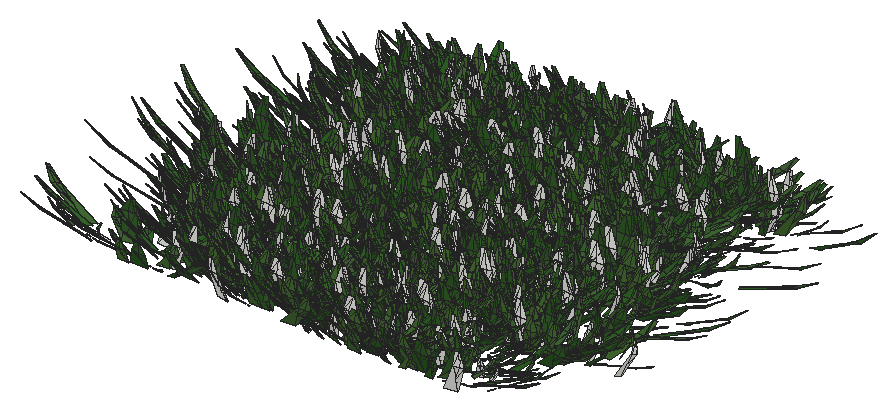
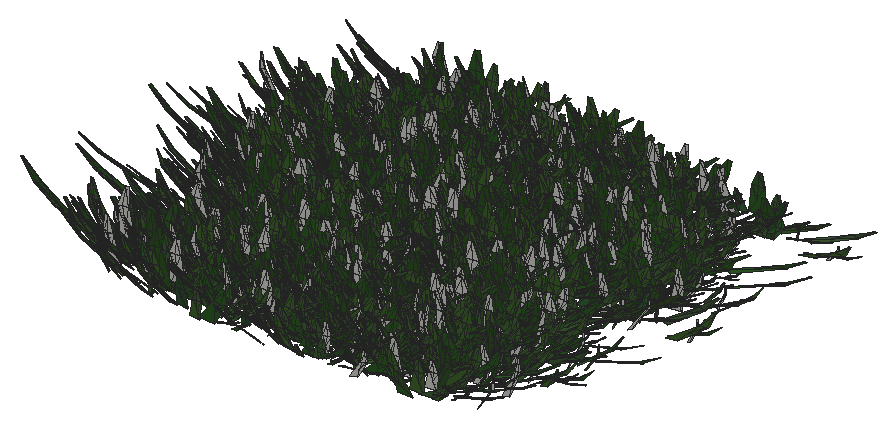
# SketchUp Ruby script. Lengths in inches.
U = 1.inch
M = Sketchup.active_model
def pt(a) = Geom::Point3d.new(a.map { |v| v * U })
def face(e, loops, mat)
  f = e.add_face(loops[0].map { |a| pt(a) })
  loops[1..].each { |l| e.add_face(l.map { |a| pt(a) }).erase! }
  f.material = f.back_material = mat if mat
  f
end
# faces: each face lists its corners as indices into pts; further lists are holes
def faces(e, pts, list, mat = nil) = list.each { |f| face(e, (f[0].is_a?(Array) ? f : [f]).map { |l| l.map { |i| pts[i] } }, mat) }
# xy, xz, yz: faces in a plane at the given z, y or x. An outline is a flat list of corners, or four numbers for a rectangle; further outlines are holes
def ring(l) = l.size == 4 ? [[l[0], l[1]], [l[2], l[1]], [l[2], l[3]], [l[0], l[3]]] : l.each_slice(2).to_a
def flat(e, list, mat, &to3) = list.each { |f| face(e, (f[0].is_a?(Array) ? f : [f]).map { |l| ring(l).map { |u, v| to3.(u, v) } }, mat) }
def xy(e, z, list, mat = nil) = flat(e, list, mat) { |x, y| [x, y, z] }
def xz(e, y, list, mat = nil) = flat(e, list, mat) { |x, z| [x, y, z] }
def yz(e, x, list, mat = nil) = flat(e, list, mat) { |y, z| [x, y, z] }
def lines(e, pts, list) = list.each { |a, b| e.add_line(pt(pts[a]), pt(pts[b])) }
# prism: a flat outline (further loops are holes) pulled along v
def prism(e, loops, v, mat = nil)
  f = face(e, loops, mat); d = Geom::Vector3d.new(v.map { |x| x * U })
  f.pushpull(f.normal.samedirection?(d) ? d.length : -d.length)
end
def box(e, o, s, mat = nil) = prism(e, [[o, [o[0] + s[0], o[1], o[2]], [o[0] + s[0], o[1] + s[1], o[2]], [o[0], o[1] + s[1], o[2]]]], [0, 0, s[2]], mat)
def at(x, y, z, deg = 0) = Geom::Transformation.translation(pt([x, y, z])) * Geom::Transformation.rotation(ORIGIN, Z_AXIS, deg.degrees)
def axes(o, x, y, z) = Geom::Transformation.new([*x, 0, *y, 0, *z, 0, *pt(o).to_a, 1])
def part(name) = M.definitions.add(name)
# library, detail: a bought-in or finely detailed component or shape, given as its bounding box
def library(name, o, s) = part(name).tap { |d| box(d.entities, o, s) }
def detail(e, o, s) = box(e.add_group.entities, o, s)
def put(e, d, t, mat = nil) = e.add_instance(d, t).tap { |i| i.material = mat if mat }
def group(e, t, mat = nil) = e.add_group.tap { |g| g.transformation = t; g.material = mat if mat }.entities
root = M.entities
M.materials.add("Material10").color = [48, 100, 38]
M.materials.add("Material3").color = [68, 110, 58]
M.materials.add("Material4").color = [48, 90, 38]
M.materials.add("Material5").color = [68, 110, 48]
M.materials.add("Material6").color = [48, 90, 48]
M.materials.add("Material7").color = [58, 110, 58]
M.materials.add("Material8").color = [58, 90, 38]
M.materials.add("Material9").color = [68, 100, 58]
c1 = part("grass00")
p = [[-0.6875,0.15,0],[-0.56,0.08,5.52],[-0.04,0.03,2.76],[0.48,-0.02,0],[0.35,-0.02,5.52],[-0.1,-0.14,5.52],
  [-0.12,0.65,8.37],[-0.42,0.65,8.37]]
faces(c1.entities,p,[[0,1,2,3],[3,2,4],[1,5,2],[5,4,2],[1,6,5],[4,5,6],[7,6,1]])
c2 = part("Group16\#1")
put(c2.entities,c1,axes([1.44,-0.61,-0.01],[0.05352,0.12609,0],[-0.10704,0.04543,0.07239],[0.06664,-0.02828,0.11628]),"Material6")
put(c2.entities,c1,axes([0.76,-0.15,-0.01],[0.04676,0.24062,0],[-0.23162,0.04501,0.06642],[0.0652,-0.01267,0.23595]),"Material3")
put(c2.entities,c1,axes([0.79,0.01,-0.01],[-0.00606,0.34651,0],[-0.34381,-0.00602,0.0432],[0.04319,0.00076,0.34386]))
put(c2.entities,c1,axes([1,0.23,-0.01],[-0.07192,0.31144,0],[-0.28722,-0.06632,0.1236],[0.12043,0.02781,0.29478]),"Material5")
put(c2.entities,c1,axes([1.66,0.77,-0.01],[-0.13828,0.29651,0],[-0.21551,-0.1005,0.22471],[0.20365,0.09498,0.23779]),"Material10")
put(c2.entities,c1,axes([0.6875,0.52,-0.01],[-0.18126,0.24051,0],[-0.22746,-0.17142,0.09788],[0.07817,0.05891,0.28481]),"Material5")
put(c2.entities,c1,axes([0.68,0.78,-0.01],[-0.215,0.18688,0],[-0.12385,-0.14248,0.21334],[0.13995,0.16101,0.18878]),"Material3")
put(c2.entities,c1,axes([0.56,1,-0.01],[-0.13756,0.07624,0],[-0.06159,-0.11112,0.0927],[0.04494,0.08108,0.12705]),"Material5")
put(c2.entities,c1,axes([0.2,0.64,-0.01],[-0.23729,0.07254,0],[-0.05711,-0.18681,0.153],[0.04473,0.14632,0.19535]),"Material10")
put(c2.entities,c1,axes([0.0625,0.72,-0.01],[-0.28874,0.02525,0],[-0.02179,-0.24916,0.14647],[0.01276,0.14591,0.25012]),"Material3")
put(c2.entities,c1,axes([-0.08,0.62,-0.01],[-0.34089,-0.04187,0],[0.03255,-0.26504,0.216],[-0.02633,0.21439,0.26703]),"Material10")
put(c2.entities,c1,axes([-0.34,0.98,-0.01],[-0.14314,-0.0493,0],[0.04397,-0.12769,0.06843],[-0.02228,0.0647,0.13505]),"Material10")
put(c2.entities,c1,axes([-0.87,1.45,-0.01],[-0.23488,-0.14114,0],[0.13761,-0.22901,0.06087],[-0.03135,0.05217,0.26717]))
put(c2.entities,c1,axes([-0.72,0.77,-0.01],[-0.14208,-0.13251,0],[0.07209,-0.0773,0.16301],[-0.11118,0.11922,0.1057]),"Material10")
put(c2.entities,c1,axes([-0.62,0.43,-0.01],[-0.14845,-0.21203,0],[0.18654,-0.13061,0.12304],[-0.10079,0.07057,0.22772]),"Material3")
put(c2.entities,c1,axes([-0.68,0.29,-0.01],[-0.13639,-0.32136,0],[0.31723,-0.13464,0.05579],[-0.05136,0.0218,0.34462]),"Material4")
put(c2.entities,c1,axes([-0.64,0.125,-0.01],[-0.0458,-0.23569,0],[0.22124,-0.043,0.08276],[-0.08124,0.01579,0.22538]),"Material7")
put(c2.entities,c1,axes([-1.6,-0.03,-0.01],[0.00576,-0.32897,0],[0.27526,0.00482,0.18018],[-0.18015,-0.00315,0.2753]),"Material5")
put(c2.entities,c1,axes([-1.36,-0.31,-0.01],[0.05718,-0.24765,0],[0.18172,0.04196,0.17267],[-0.16825,-0.03885,0.1865]),"Material10")
put(c2.entities,c1,axes([-1.54,-0.72,-0.01],[0.06537,-0.14017,0],[0.13555,0.06321,0.03939],[-0.0357,-0.01665,0.14956]))
put(c2.entities,c1,axes([-1.19,-0.9,-0.01],[0.09597,-0.12735,0],[0.11214,0.08451,0.07557],[-0.06035,-0.04548,0.14042]),"Material9")
put(c2.entities,c1,axes([-0.47,-0.54,-0.01],[0.11588,-0.10072,0],[0.0618,0.0711,0.12124],[-0.07953,-0.0915,0.0942]))
put(c2.entities,c1,axes([-0.47,-0.84,-0.01],[0.11927,-0.0661,0],[0.06603,0.11913,0.00646],[-0.00313,-0.00565,0.13621]),"Material5")
put(c2.entities,c1,axes([-0.38,-1.24,-0.01],[0.28037,-0.08571,0],[0.0618,0.20215,0.20315],[-0.05939,-0.19428,0.21139]),"Material9")
put(c2.entities,c1,axes([-0.06,-0.66,-0.01],[0.22719,-0.01987,0],[0.01247,0.14255,0.17758],[-0.01547,-0.17691,0.1431]),"Material8")
put(c2.entities,c1,axes([0.11,-0.89,-0.01],[0.14882,0.01828,0],[-0.01058,0.08611,0.12229],[0.01491,-0.12138,0.08676]),"Material6")
put(c2.entities,c1,axes([0.25,-0.72,-0.01],[0.20481,0.07053,0],[-0.06206,0.18022,0.10291],[0.03351,-0.0973,0.1906]),"Material6")
put(c2.entities,c1,axes([0.85,-1.42,-0.01],[0.16481,0.09904,0],[-0.09472,0.15762,0.05616],[0.02893,-0.04814,0.18389]),"Material5")
put(c2.entities,c1,axes([1.01,-1.09,-0.01],[0.21858,0.20385,0],[-0.17495,0.1876,0.15339],[0.10462,-0.11218,0.25652]),"Material10")
put(c2.entities,c1,axes([1.01,-0.71,-0.01],[0.08733,0.12473,0],[-0.06445,0.04512,0.13037],[0.1068,-0.07477,0.07867]),"Material6")
c3 = part("Group15\#1")
put(c3.entities,c2,at(0,0,0))
c4 = part("3darcstudiotree_grass00\#1")
put(c4.entities,c3,at(0,0,0))
put(root,c4,axes([56.96,43.7,7.6],[4.17584,-0.76775,0],[2.82757,0.96121,-0.02397],[0.06306,0.02144,1.32443]))
put(root,c4,axes([56.96,61.42,7.6],[4.18652,-0.74489,0],[2.19035,0.7694,-0.02041],[0.09799,0.03442,1.95445]))
put(root,c4,axes([56.8,57.02,7.6],[4.0539,0.02185,0],[-0.08547,0.99116,-0.0399],[-0.00654,0.07588,1.8861]))
put(root,c4,axes([59.84,71.05,7.6],[-1.7872,-0.89941,0],[4.01851,-0.49907,-0.01655],[0.09453,-0.01174,1.78815]))
put(root,c4,axes([61.12,74.68,7.6],[-3.91628,-0.80857,0],[3.0662,-0.92819,-0.02974],[0.08498,-0.02572,1.35064]))
put(root,c4,axes([60.84,55.08,7.6],[-0.87255,-1.13865,0],[3.68469,-0.17647,-0.01579],[0.09603,-0.0046,1.45182]))
put(root,c4,axes([61.39,52.02,7.6],[-4.92325,-0.27664,0],[0.91141,-1.01375,-0.03373],[0.03797,-0.04223,1.33323]))
put(root,c4,axes([61.31,53.55,7.6],[-5.12565,0.19811,0],[-0.59233,-0.95782,-0.03554],[-0.04116,-0.06655,1.83631]))
put(root,c4,axes([59.92,58.05,7.6],[-0.11297,1.08035,0],[-4.48718,-0.02933,-0.03889],[-0.20921,-0.00137,1.50954]))
put(root,c4,axes([60.81,56.58,7.6],[-3.61171,0.88239,0],[-2.76709,-0.70787,-0.01484],[-0.07769,-0.01988,1.85373]))
put(root,c4,axes([60.95,61.21,7.6],[2.72646,-0.79563,0],[3.21066,0.68764,-0.00664],[0.02825,0.00605,1.48048]))
put(root,c4,axes([59.96,72.58,7.6],[0.71242,1.197,0],[-3.75762,0.13978,-0.01524],[-0.1206,0.00449,1.90022]))
put(root,c4,axes([61.17,68.53,7.6],[-3.36041,0.90799,0],[-3.17072,-0.73341,-0.0352],[-0.15551,-0.03597,1.62511]))
put(root,c4,axes([60.63,77.82,7.6],[2.92569,0.54408,0],[-2.20569,0.74129,-0.0148],[-0.07382,0.02481,1.93047]))
put(root,c4,axes([62.53,64.34,7.6],[-1.3197,-0.88454,0],[4.35554,-0.40614,-0.0406],[0.24185,-0.02255,1.84742]))
put(root,c4,axes([61.6,49.72,7.6],[-0.61826,0.98554,0],[-3.83572,-0.15039,-0.01794],[-0.11657,-0.00457,1.59592]))
put(root,c4,axes([61.65,76.46,7.6],[4.34755,0.01968,0],[-0.0883,1.21931,-0.04973],[-0.00561,0.07747,1.89995]))
put(root,c4,axes([61.58,63.57,7.6],[2.15023,1.14351,0],[-3.90551,0.45899,-0.03464],[-0.20705,0.02433,1.78143]))
put(root,c4,axes([62.01,81.66,7.6],[1.34979,0.94972,0],[-3.68739,0.32754,-0.0026],[-0.01469,0.00131,1.46428]))
put(root,c4,axes([64.05,44.89,7.6],[-2.47748,-1.01613,0],[3.676,-0.56016,-0.05337],[0.25605,-0.03902,1.5119]))
put(root,c4,axes([64.21,68,7.6],[-2.66833,-0.96931,0],[3.87821,-0.66725,-0.05298],[0.21893,-0.03767,1.4759]))
put(root,c4,axes([63.56,59.68,7.6],[2.30666,-1.0875,0],[4.46305,0.59165,-0.05067],[0.21491,0.02849,1.51576]))
put(root,c4,axes([63.46,46.125,7.6],[2.28163,-1.10876,0],[3.45513,0.44438,-0.03693],[0.24001,0.03087,1.77491]))
put(root,c4,axes([62.41,50.92,7.6],[0.86518,1.01256,0],[-4.67116,0.24945,-0.00171],[-0.00978,0.00052,1.74655]))
put(root,c4,axes([64.29,66.44,7.6],[1.85636,-0.87548,0],[4.2252,0.55994,-0.01977],[0.10435,0.01383,1.78562]))
put(root,c4,axes([63.04,47.43,7.6],[3.65118,0.22835,0],[-1.21465,1.21387,-0.00744],[-0.00809,0.00808,1.4009]))
put(root,c4,axes([63.55,79.6,7.6],[3.69854,-0.02221,0],[0.11187,1.16446,-0.04057],[0.00448,0.0466,1.33829]))
put(root,c4,axes([64.26,73.52,7.6],[1.29993,0.864,0],[-3.89937,0.36667,-0.04913],[-0.3212,0.0302,1.81865]))
put(root,c4,axes([66.06,77.99,7.6],[-4.57324,0.06463,0],[-0.23944,-1.05899,-0.00256],[-0.00093,-0.0041,1.70382]))
put(root,c4,axes([66.87,73.17,7.6],[-0.89657,-1.00818,0],[4.16611,-0.23156,-0.01455],[0.07266,-0.00404,1.36448]))
put(root,c4,axes([67.1,50.92,7.6],[-4.48956,-0.10603,0],[0.4036,-1.06805,-0.03137],[0.01455,-0.03851,1.3228]))
put(root,c4,axes([66.5,63.01,7.6],[-3.51738,0.88979,0],[-2.84475,-0.70284,-0.03007],[-0.16867,-0.04167,1.97134]))
put(root,c4,axes([67.59,56.49,7.6],[-1.66366,-1.09388,0],[4.81129,-0.45734,-0.02869],[0.11735,-0.01115,1.40786]))
put(root,c4,axes([67.51,76.45,7.6],[-3.48279,-0.87064,0],[3.22991,-0.80753,-0.05204],[0.22842,-0.05711,1.77215]))
put(root,c4,axes([66.46,67.875,7.6],[3.6556,-0.00646,0],[0.03301,1.16694,-0.0442],[0.00143,0.05063,1.33678]))
put(root,c4,axes([67.78,79.21,7.6],[-0.76209,-0.8955,0],[4.21088,-0.22397,-0.04713],[0.27128,-0.01443,1.58351]))
put(root,c4,axes([68.01,46.2,7.6],[-4.62143,0.243,0],[-0.94962,-1.12878,-0.01674],[-0.02169,-0.02578,1.81501]))
put(root,c4,axes([67.32,59.51,7.6],[-1.86129,1.04113,0],[-3.56127,-0.39792,-0.0353],[-0.23679,-0.02646,1.79152]))
put(root,c4,axes([66.67,69.09,7.6],[-0.25494,0.97633,0],[-4.14,-0.06757,-0.01044],[-0.06049,-0.00099,1.50484]))
put(root,c4,axes([67.27,58.78,7.6],[-1.81241,0.85441,0],[-3.27922,-0.43475,-0.02105],[-0.15086,-0.02,1.88169]))
put(root,c4,axes([66.54,49.53,7.6],[3.58871,0.50463,0],[-2.17344,0.96603,-0.00275],[-0.00669,0.00297,1.37565]))
put(root,c4,axes([68.67,52,7.6],[-3.15251,-0.61197,0],[3.07523,-0.99011,-0.06125],[0.16311,-0.05251,1.36064]))
put(root,c4,axes([68.18,55.48,7.6],[0.12937,-1.28679,0],[4.29461,0.02699,-0.05528],[0.32895,0.00207,1.59813]))
put(root,c4,axes([67.29,70.44,7.6],[-1.95389,0.95896,0],[-4.54088,-0.57825,-0.01882],[-0.07855,-0.01,1.49212]))
put(root,c4,axes([69.26,74.9,7.6],[0.30161,-1.10509,0],[5.10821,0.08714,-0.02398],[0.09779,0.00167,1.30813]))
put(root,c4,axes([68.79,80.89,7.6],[-4.48167,0.42231,0],[-1.44453,-0.9581,-0.00238],[-0.00433,-0.00287,1.31717]))
put(root,c4,axes([69.67,61.87,7.6],[-1.21535,-0.91451,0],[3.60544,-0.29947,-0.00285],[0.02203,-0.00183,1.93438]))
put(root,c4,axes([69.64,54.01,7.6],[-2.37468,-0.98502,0],[3.18628,-0.48009,-0.03107],[0.19051,-0.0287,1.66455]))
put(root,c4,axes([69.89,65.03,7.6],[-4.21878,-0.13998,0],[0.64353,-1.21222,-0.01228],[0.00866,-0.0163,1.63767]))
put(root,c4,axes([69.99,44.8,7.6],[0.48505,-1.08337,0],[4.27123,0.11952,-0.04376],[0.24596,0.00688,1.51939]))
put(root,c4,axes([69.44,72.58,7.6],[-2.73895,0.66336,0],[-3.26902,-0.84359,-0.02879],[-0.12001,-0.03097,1.7592]))
put(root,c4,axes([69.56,43.48,7.6],[-2.4816,0.92551,0],[-3.41349,-0.57204,-0.02214],[-0.11703,-0.01961,1.63462]))
put(root,c4,axes([69.94,65.85,7.6],[-1.82662,0.77889,0],[-3.91562,-0.57392,-0.01566],[-0.07709,-0.0113,1.61828]))
put(root,c4,axes([70.05,47.76,7.6],[4.05704,-0.60104,0],[1.84911,0.7801,-0.02001],[0.07729,0.03261,1.71774]))
put(root,c4,axes([72.03,78.51,7.6],[-3.56139,-0.59682,0],[2.57727,-0.96121,-0.05337],[0.16285,-0.06074,1.58535]))
put(root,c4,axes([73.2,80.16,7.6],[-3.83504,-0.49614,0],[2.03803,-0.98459,-0.02021],[0.06424,-0.03103,1.91641]))
put(root,c4,axes([73.5,75.28,7.6],[0.25783,-1.11098,0],[4.27668,0.06203,-0.02273],[0.12742,0.00185,1.50351]))
put(root,c4,axes([72.76,73.91,7.6],[4.62804,-0.23272,0],[0.89278,1.10968,-0.02659],[0.02814,0.03498,1.51897]))
put(root,c4,axes([74.79,65.09,7.6],[-4.56641,-0.61307,0],[2.03224,-0.94607,-0.02099],[0.05514,-0.02567,1.49075]))
put(root,c4,axes([72.77,82.41,7.6],[3.22508,0.4199,0],[-2.23997,1.07528,-0.0178],[-0.0355,0.01704,1.30843]))
put(root,c4,axes([73.95,52.71,7.6],[2.46228,-0.71132,0],[3.57586,0.77364,-0.03846],[0.1554,0.03362,1.57923]))
put(root,c4,axes([74.77,65.71,7.6],[-2.12409,-0.80452,0],[3.07899,-0.50807,-0.03406],[0.21345,-0.03522,1.73123]))
put(root,c4,axes([75.16,51.05,7.6],[-2.37888,-1.01371,0],[3.74365,-0.54908,-0.03431],[0.16796,-0.02463,1.53951]))
put(root,c4,axes([74.43,59.87,7.6],[2.88746,-1.01127,0],[4.01064,0.71572,-0.04124],[0.17013,0.03036,1.56101]))
put(root,c4,axes([74.78,69.02,7.6],[0.65857,-1.17921,0],[3.67761,0.12837,-0.0384],[0.25113,0.00877,1.53253]))
put(root,c4,axes([73.88,58.86,7.6],[3.72974,0.07459,0],[-0.38183,1.19325,-0.00093],[-0.00033,0.00104,1.35201]))
put(root,c4,axes([73.57,49.52,7.6],[4.3834,0.50633,0],[-1.68665,0.91261,-0.00765],[-0.01741,0.00942,1.36419]))
put(root,c4,axes([75.57,62.7,7.6],[0.55792,-1.05016,0],[4.92434,0.16351,-0.03191],[0.17517,0.00582,1.71939]))
put(root,c4,axes([75.85,46.43,7.6],[-4.56826,-0.36259,0],[1.35513,-1.06708,-0.0262],[0.03858,-0.03038,1.36239]))
put(root,c4,axes([73.64,76.53,7.6],[4.02014,0.68076,0],[-2.86441,1.05721,-0.02464],[-0.08583,0.03168,1.98292]))
put(root,c4,axes([75.84,54.88,7.6],[-3.83129,-0.35772,0],[1.74028,-1.16494,-0.03885],[0.07795,-0.05218,1.78292]))
put(root,c4,axes([73.95,60.98,7.6],[-0.31476,0.91274,0],[-4.84329,-0.10439,-0.00545],[-0.03468,-0.00075,1.93955]))
put(root,c4,axes([74.96,70.41,7.6],[-1.66993,0.87259,0],[-3.97117,-0.47499,-0.02774],[-0.12868,-0.01539,1.41462]))
put(root,c4,axes([74.14,71.76,7.6],[3.65221,0.81587,0],[-2.94048,0.82269,-0.00121],[-0.00437,0.00122,1.48985]))
put(root,c4,axes([76.31,56.66,7.6],[-4.23214,-0.05547,0],[0.1952,-0.93083,-0.00586],[0.00226,-0.01076,1.71352]))
put(root,c4,axes([74.75,53.93,7.6],[0.83957,1.19196,0],[-3.66821,0.16148,-0.02162],[-0.1209,0.00532,1.32159]))
put(root,c4,axes([75.125,81.15,7.6],[3.80473,0.13574,0],[-0.67195,1.17716,-0.03434],[-0.02787,0.04883,1.70799]))
put(root,c4,axes([74.85,67.64,7.6],[4.29167,0.73108,0],[-2.5905,0.95044,-0.06012],[-0.15898,0.05833,1.3502]))
put(root,c4,axes([75.62,44.28,7.6],[0.81792,0.98803,0],[-4.75058,0.24579,-0.00233],[-0.01332,0.00069,1.77271]))
put(root,c4,axes([76.125,48.3,7.6],[3.79999,0.06244,0],[-0.29859,1.1358,-0.01423],[-0.00601,0.02286,1.83161]))
put(root,c4,axes([78.59,46.7,7.6],[-4.93822,-0.11046,0],[0.42261,-1.18087,-0.03473],[0.01792,-0.05006,1.7157]))
put(root,c4,axes([78.98,72.39,7.6],[0.15957,-0.94034,0],[4.98466,0.05287,-0.04061],[0.22246,0.00236,1.70991]))
put(root,c4,axes([79.33,56.54,7.6],[-1.41294,-1.10212,0],[4.32228,-0.34633,-0.03893],[0.21471,-0.0172,1.64312]))
put(root,c4,axes([79.62,58.42,7.6],[-3.69312,-0.8813,0],[3.34955,-0.87728,-0.04863],[0.21671,-0.05676,1.95701]))
put(root,c4,axes([79.4,44.32,7.6],[-0.87663,-1.01395,0],[4.66847,-0.25226,-0.06129],[0.26842,-0.0145,1.3376]))
put(root,c4,axes([78.57,76.83,7.6],[3.5325,-0.69831,0],[2.94663,0.93162,-0.01988],[0.08154,0.02578,1.96304]))
put(root,c4,axes([79.33,64.6875,7.6],[0.77857,-0.99525,0],[5.0673,0.24776,-0.06032],[0.25875,0.01265,1.41053]))
put(root,c4,axes([79.375,60.26,7.6],[-3.85062,-0.01072,0],[0.0412,-0.92486,-0.02017],[0.00173,-0.03873,1.77597]))
put(root,c4,axes([79.98,47.7,7.6],[-2.58333,-1.04048,0],[3.69668,-0.57364,-0.02087],[0.10332,-0.01603,1.58468]))
put(root,c4,axes([79.72,78.48,7.6],[-3.948,-0.1076,0],[0.50589,-1.16017,-0.01401],[0.009,-0.02065,1.72979]))
put(root,c4,axes([80.14,74.1875,7.6],[-5.08538,0.01363,0],[-0.0515,-1.20054,-0.01941],[-0.00134,-0.03118,1.92834]))
put(root,c4,axes([78.93,70.21,7.6],[4.17924,-0.09662,0],[0.4087,1.10487,-0.00914],[0.00578,0.01563,1.90465]))
put(root,c4,axes([79.02,51.21,7.6],[2.55931,1.04661,0],[-3.2663,0.4992,-0.02868],[-0.15491,0.02367,1.51486]))
put(root,c4,axes([81.02,67.53,7.6],[-0.89831,-1.0989,0],[4.77812,-0.24412,-0.03636],[0.19134,-0.00978,1.63697]))
put(root,c4,axes([80.08,80.67,7.6],[-2.18401,1.00403,0],[-3.62225,-0.49246,-0.03157],[-0.1939,-0.02636,1.80167]))
put(root,c4,axes([79.64,43.24,7.6],[3.60668,0.39506,0],[-2.04442,1.16653,-0.0492],[-0.09575,0.05464,1.54416]))
put(root,c4,axes([80.125,75.3125,7.6],[4.80917,-0.20992,0],[0.88931,1.27332,-0.04063],[0.03159,0.04524,1.46079]))
put(root,c4,axes([81.94,49.78,7.6],[0.74314,-1.27426,0],[5.01119,0.18265,-0.00277],[0.01296,0.00047,1.49508]))
put(root,c4,axes([80.31,65.49,7.6],[4.05871,-0.05513,0],[0.21483,0.98855,-0.02262],[0.008,0.03681,1.6131]))
put(root,c4,axes([80.45,52.42,7.6],[2.41461,0.82437,0],[-3.20063,0.58592,-0.01948],[-0.10927,0.02,1.72408]))
put(root,c4,axes([82.16,61.64,7.6],[-4.13654,0.57707,0],[-2.0044,-0.898,-0.03544],[-0.10461,-0.04686,1.55733]))
put(root,c4,axes([82.26,54.96,7.6],[2.18961,-0.72887,0],[3.37602,0.63387,-0.00267],[0.01513,0.00284,1.87177]))
put(root,c4,axes([82.45,63.35,7.6],[-4.20241,0.23168,0],[-1.01309,-1.14851,-0.02531],[-0.03283,-0.03722,1.77094]))
put(root,c4,axes([81.0625,54.05,7.6],[3.66493,0.77131,0],[-3.09992,0.92059,-0.01247],[-0.04973,0.01477,1.86292]))
put(root,c4,axes([82.37,79.28,7.6],[4.71809,-0.16737,0],[0.67524,1.18967,-0.05794],[0.04945,0.08711,1.82474]))
put(root,c4,axes([84.26,59.45,7.6],[-3.89812,-0.79774,0],[2.64275,-0.80711,-0.04086],[0.17451,-0.0533,1.75811]))
put(root,c4,axes([82.23,69.47,7.6],[0.07283,1.03714,0],[-5.06058,0.02221,-0.00579],[-0.03358,0.00015,1.83497]))
put(root,c4,axes([84.59,52.74,7.6],[-0.48105,-1.08782,0],[3.72041,-0.10283,-0.00454],[0.03276,-0.00091,1.6986]))
put(root,c4,axes([84.96,48.88,7.6],[-2.15929,-1.00318,0],[4.02891,-0.542,-0.04084],[0.19903,-0.02677,1.58232]))
put(root,c4,axes([84.76,47.96,7.6],[-3.84728,0.08343,0],[-0.38404,-1.1069,-0.04163],[-0.02453,-0.07069,1.89396]))
put(root,c4,axes([85.54,77.22,7.6],[-1.13756,-1.10329,0],[4.36364,-0.2812,-0.01269],[0.0739,-0.00476,1.69312]))
put(root,c4,axes([84.05,69.4,7.6],[-1.05633,0.97001,0],[-4.93574,-0.33594,-0.06593],[-0.31871,-0.02169,1.60187]))
put(root,c4,axes([85.59,58.76,7.6],[-1.37062,-0.86535,0],[3.38403,-0.33499,-0.01359],[0.09291,-0.0092,1.67314]))
put(root,c4,axes([85.29,82.5625,7.6],[-4.71082,0.41428,0],[-1.209,-0.85923,-0.00518],[-0.01407,-0.01,1.86492]))
put(root,c4,axes([84.94,63.23,7.6],[-3.26227,0.95653,0],[-3.0473,-0.64955,-0.01811],[-0.0716,-0.01526,1.30017]))
put(root,c4,axes([85.93,43.2,7.6],[-4.67365,-0.16733,0],[0.64986,-1.13441,-0.00988],[0.00864,-0.01508,1.76639]))
put(root,c4,axes([85.14,44.64,7.6],[2.69465,-0.83089,0],[3.37548,0.68418,-0.02965],[0.1163,0.02357,1.3715]))
put(root,c4,axes([86.75,67.375,7.6],[-4.67486,-0.01007,0],[0.0413,-1.19802,-0.00939],[0.00051,-0.01491,1.9024]))
put(root,c4,axes([86.37,75.52,7.6],[2.36561,-1.09039,0],[3.75477,0.50912,-0.01711],[0.08085,0.01096,1.43496]))
put(root,c4,axes([85.23,55.06,7.6],[3.54618,0.29573,0],[-1.39586,1.04613,-0.00681],[-0.0149,0.01117,1.90695]))
put(root,c4,axes([87.24,66.21,7.6],[0.13363,-1.19424,0],[4.75685,0.03327,-0.00421],[0.02569,0.00018,1.81536]))
put(root,c4,axes([85.58,53.6875,7.6],[3.3147,0.39945,0],[-1.62402,0.84226,-0.04063],[-0.11562,0.05996,1.53169]))
put(root,c4,axes([85.72,50.375,7.6],[-0.8661,0.95762,0],[-4.99229,-0.2822,-0.04071],[-0.17859,-0.0101,1.43871]))
put(root,c4,axes([86.22,71.91,7.6],[-1.64669,0.8129,0],[-3.86386,-0.48919,-0.03106],[-0.13559,-0.01717,1.32443]))
put(root,c4,axes([86.8125,70.92,7.6],[-0.66417,1.24214,0],[-3.94693,-0.1319,-0.04319],[-0.32199,-0.01076,1.87209]))
put(root,c4,axes([87.98,79.15,7.6],[-2.88434,-1.08053,0],[3.30861,-0.55199,-0.04802],[0.27291,-0.04553,1.69851]))
put(root,c4,axes([88.12,78.66,7.6],[-2.43926,-0.75546,0],[3.00839,-0.6071,-0.02577],[0.12993,-0.02622,1.56591]))
put(root,c4,axes([88.26,64.375,7.6],[1.40965,-1.22459,0],[4.89499,0.35217,-0.04991],[0.29274,0.02106,1.94306]))
put(root,c4,axes([87.29,57.13,7.6],[4.02811,0.14495,0],[-0.62755,1.08997,-0.04848],[-0.03789,0.0658,1.51023]))
put(root,c4,axes([88.5,61.79,7.6],[1.97657,-1.09478,0],[4.53961,0.51226,-0.03311],[0.18515,0.02089,1.9099]))
put(root,c4,axes([88.33,73.46,7.6],[3.73189,-0.79039,0],[3.05525,0.9016,-0.02128],[0.07472,0.02205,1.60475]))
put(root,c4,axes([87.61,80.85,7.6],[3.02072,0.55371,0],[-2.49309,0.85005,-0.01003],[-0.03081,0.0105,1.36834]))
put(root,c4,axes([88.43,46.14,7.6],[-0.05036,0.9122,0],[-4.03492,-0.01392,-0.02407],[-0.14251,-0.00049,1.49365]))
put(root,c4,axes([91.22,51.13,7.6],[0.09023,-0.92419,0],[3.99755,0.02439,-0.00377],[0.02513,0.00015,1.66719]))
put(root,c4,axes([90.74,64,7.6],[-2.09892,1.15231,0],[-3.29486,-0.3751,-0.04508],[-0.24035,-0.02736,1.32557]))
put(root,c4,axes([90.51,69.08,7.6],[4.49325,-0.21308,0],[0.91825,1.21019,-0.00778],[0.00669,0.00882,1.42033]))
put(root,c4,axes([90.94,57.33,7.6],[-2.22405,0.97958,0],[-4.34161,-0.61608,-0.03094],[-0.11665,-0.01655,1.35284]))
put(root,c4,axes([90.74,58.23,7.6],[4.35501,-0.07003,0],[0.31999,1.24382,-0.04097],[0.01403,0.05455,1.66267]))
put(root,c4,axes([91.47,62.52,7.6],[3.24444,-0.662,0],[2.42795,0.74371,-0.03627],[0.18046,0.05528,1.88825]))
put(root,c4,axes([92.74,52.18,7.6],[-2.89851,-0.94467,0],[3.35055,-0.64252,-0.03114],[0.17556,-0.03367,1.87535]))
put(root,c4,axes([92.1,79.28,7.6],[3.0338,-0.77588,0],[3.0604,0.74791,-0.00015],[0.00078,0.00019,1.98495]))
put(root,c4,axes([91.13,54.22,7.6],[1.49753,0.88815,0],[-4.28846,0.45193,-0.04214],[-0.25848,0.02724,1.93625]))
